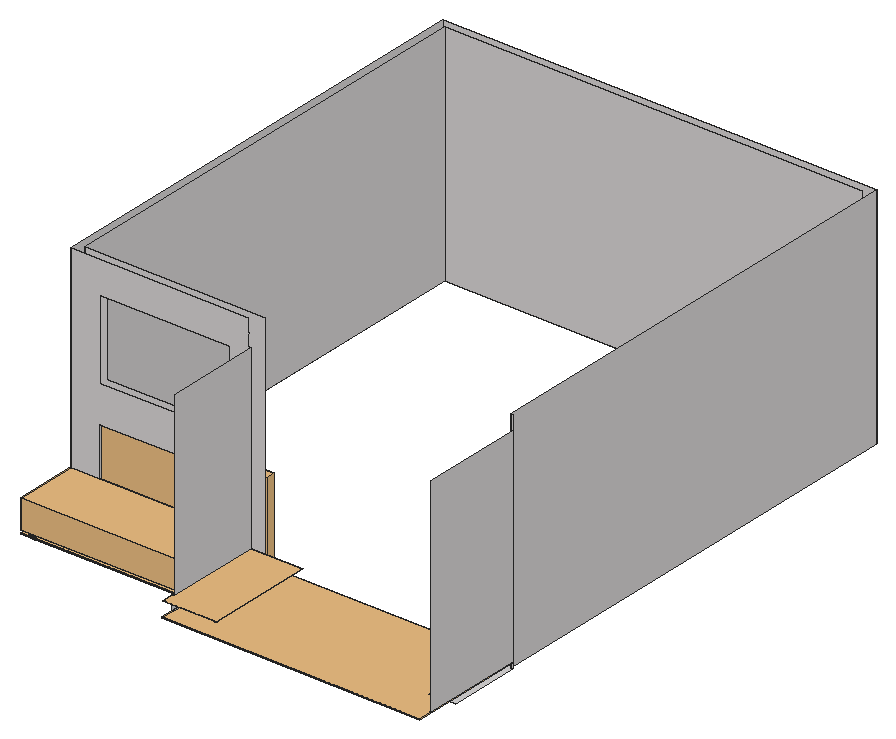
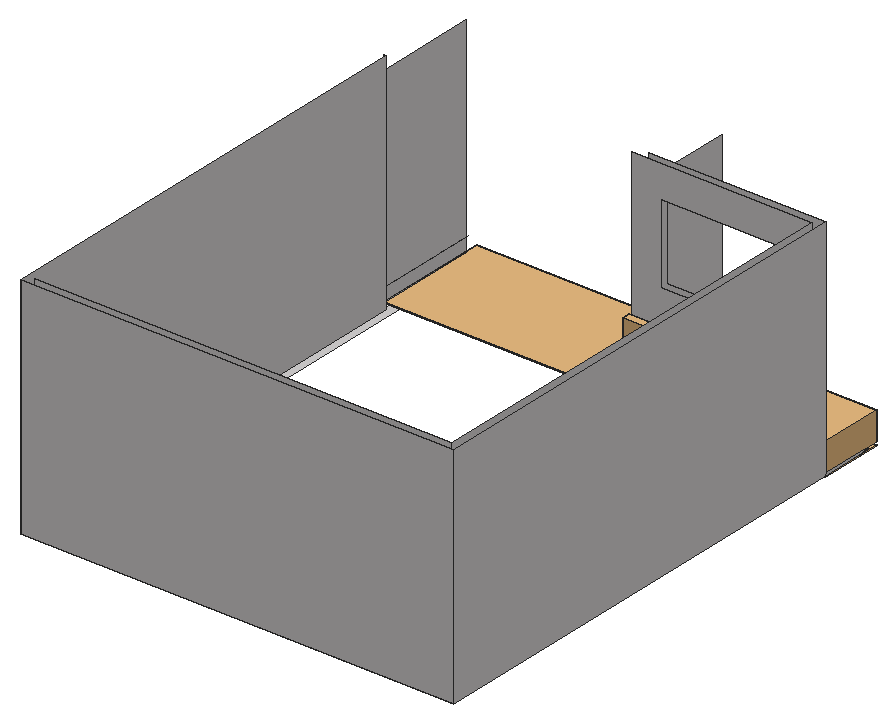
# SketchUp Ruby script. Lengths in inches.
U = 1.inch
M = Sketchup.active_model
def pt(a) = Geom::Point3d.new(a.map { |v| v * U })
def face(e, loops, mat)
  f = e.add_face(loops[0].map { |a| pt(a) })
  loops[1..].each { |l| e.add_face(l.map { |a| pt(a) }).erase! }
  f.material = f.back_material = mat if mat
  f
end
# faces: each face lists its corners as indices into pts; further lists are holes
def faces(e, pts, list, mat = nil) = list.each { |f| face(e, (f[0].is_a?(Array) ? f : [f]).map { |l| l.map { |i| pts[i] } }, mat) }
# xy, xz, yz: faces in a plane at the given z, y or x. An outline is a flat list of corners, or four numbers for a rectangle; further outlines are holes
def ring(l) = l.size == 4 ? [[l[0], l[1]], [l[2], l[1]], [l[2], l[3]], [l[0], l[3]]] : l.each_slice(2).to_a
def flat(e, list, mat, &to3) = list.each { |f| face(e, (f[0].is_a?(Array) ? f : [f]).map { |l| ring(l).map { |u, v| to3.(u, v) } }, mat) }
def xy(e, z, list, mat = nil) = flat(e, list, mat) { |x, y| [x, y, z] }
def xz(e, y, list, mat = nil) = flat(e, list, mat) { |x, z| [x, y, z] }
def yz(e, x, list, mat = nil) = flat(e, list, mat) { |y, z| [x, y, z] }
def lines(e, pts, list) = list.each { |a, b| e.add_line(pt(pts[a]), pt(pts[b])) }
# prism: a flat outline (further loops are holes) pulled along v
def prism(e, loops, v, mat = nil)
  f = face(e, loops, mat); d = Geom::Vector3d.new(v.map { |x| x * U })
  f.pushpull(f.normal.samedirection?(d) ? d.length : -d.length)
end
def box(e, o, s, mat = nil) = prism(e, [[o, [o[0] + s[0], o[1], o[2]], [o[0] + s[0], o[1] + s[1], o[2]], [o[0], o[1] + s[1], o[2]]]], [0, 0, s[2]], mat)
def at(x, y, z, deg = 0) = Geom::Transformation.translation(pt([x, y, z])) * Geom::Transformation.rotation(ORIGIN, Z_AXIS, deg.degrees)
def axes(o, x, y, z) = Geom::Transformation.new([*x, 0, *y, 0, *z, 0, *pt(o).to_a, 1])
def part(name) = M.definitions.add(name)
# library, detail: a bought-in or finely detailed component or shape, given as its bounding box
def library(name, o, s) = part(name).tap { |d| box(d.entities, o, s) }
def detail(e, o, s) = box(e.add_group.entities, o, s)
def put(e, d, t, mat = nil) = e.add_instance(d, t).tap { |i| i.material = mat if mat }
def group(e, t, mat = nil) = e.add_group.tap { |g| g.transformation = t; g.material = mat if mat }.entities
root = M.entities
M.materials.add("Outer Light - 1").color = [251, 216, 141]
M.materials.add("T METAL").color = [42, 41, 39]
M.materials.add("[Marble Carrara Floor Tile]").color = [204, 208, 219]
M.materials.add("[Quartz Light Brown]").color = [215, 212, 212]
c1 = library("Group\#10",[0,0,0],[61.75,122.25,0.25])
c2 = library("Group\#15",[-0.75,-0.75,0],[293.5,131.75,1])
c3 = library("Group\#20",[-0.5,-0.5,0],[204,72,1])
c4 = library("Group\#23",[0,0,0],[201,72,32])
c5 = library("Glass Door Sliding Door 4 Panel on 2 Tracks _ Model by Pooh",[0,0,0],[157.59,4.01,102.67])
c6 = library("Garniza_zaclona",[1.52,0,0],[127.96,8.15,78.72])
xy(root,125,[[17.76,194,201,194,201,194.5,17.77,194.5,17.54,194.51,17.3125,194.51,17.08,194.52,16.86,194.54,16.625,194.55,16.4,194.57,16.17,194.6,15.94,194.62,15.72,194.65,15.49,194.68,15.26,194.72,15.04,194.75,14.8125,194.79,14.59,194.84,14.36,194.88,14.14,194.93,13.91,194.98,13.03,195.22,12.8125,195.29,12.59,195.36,12.16,195.5,11.94,195.58,11.73,195.66,11.52,195.75,11.3,195.83,10.88,196.01,10.67,196.11,10.47,196.2,10.26,196.3,10.06,196.41,9.85,196.51,9.25,196.84,9.05,196.96,8.86,197.08,8.66,197.2,8.47,197.32,7.71,197.84,6.99,198.4,6.81,198.55,6.63,198.69,6.29,198.99,5.95,199.31,5.79,199.46,5.46,199.79,5.31,199.95,4.99,200.29,4.69,200.63,4.55,200.81,4.4,200.99,3.84,201.71,3.32,202.47,3.2,202.66,3.08,202.86,2.96,203.05,2.84,203.25,2.51,203.85,2.41,204.06,2.3,204.26,2.2,204.47,2.11,204.67,2.01,204.88,1.83,205.3,1.75,205.52,1.66,205.73,1.58,205.94,1.5,206.16,1.36,206.59,1.29,206.8125,1.22,207.03,0.98,207.91,0.93,208.14,0.88,208.36,0.84,208.59,0.79,208.8125,0.75,209.04,0.72,209.26,0.68,209.49,0.65,209.72,0.62,209.94,0.6,210.17,0.57,210.4,0.55,210.625,0.54,210.86,0.52,211.08,0.51,211.3125,0.51,211.54,0.5,211.77,0.5,266,0,266,0,211.76,0.01,211.53,0.01,211.29,0.02,211.06,0.04,210.82,0.06,210.59,0.08,210.35,0.1,210.12,0.125,209.88,0.15,209.65,0.1875,209.42,0.22,209.18,0.3,208.72,0.35,208.49,0.39,208.26,0.44,208.03,0.5,207.8,0.55,207.57,0.61,207.34,0.68,207.11,0.74,206.89,0.81,206.66,0.88,206.4375,0.96,206.21,1.03,205.99,1.11,205.77,1.2,205.55,1.28,205.33,1.46,204.89,1.56,204.68,1.65,204.46,1.75,204.25,1.86,204.04,1.96,203.83,2.18,203.41,2.3,203.2,2.41,203,2.65,202.6,2.78,202.39,2.9,202.2,3.03,202,3.17,201.8,3.3,201.61,3.4375,201.42,3.58,201.23,3.72,201.04,3.86,200.86,4.01,200.67,4.16,200.49,4.3125,200.31,4.47,200.13,4.625,199.96,4.78,199.78,4.94,199.61,5.11,199.44,5.27,199.27,5.44,199.11,5.61,198.94,5.78,198.78,5.96,198.625,6.13,198.47,6.31,198.3125,6.49,198.16,6.67,198.01,6.86,197.86,7.04,197.72,7.23,197.58,7.42,197.4375,7.61,197.3,7.8,197.17,8,197.03,8.2,196.9,8.39,196.78,8.6,196.65,9,196.41,9.2,196.3,9.41,196.18,9.83,195.96,10.04,195.86,10.25,195.75,10.46,195.65,10.68,195.56,10.89,195.46,11.33,195.28,11.55,195.2,11.77,195.11,11.99,195.03,12.21,194.96,12.4375,194.88,12.66,194.81,12.89,194.74,13.11,194.68,13.34,194.61,13.57,194.55,13.8,194.5,14.03,194.44,14.26,194.39,14.49,194.35,14.72,194.3,15.18,194.22,15.42,194.1875,15.65,194.15,15.88,194.125,16.12,194.1,16.35,194.08,16.59,194.06,16.82,194.04,17.06,194.02,17.29,194.01,17.53,194.01]],"[Quartz Light Brown]")
xy(root,126,[[0,266,3,794]],"[Marble Carrara Floor Tile]")
xy(root,126,[[17.76,194,17.53,194.01,17.29,194.01,17.06,194.02,16.82,194.04,16.59,194.06,16.35,194.08,16.12,194.1,15.88,194.125,15.65,194.15,15.42,194.1875,15.18,194.22,14.72,194.3,14.49,194.35,14.26,194.39,14.03,194.44,13.8,194.5,13.57,194.55,13.34,194.61,13.11,194.68,12.89,194.74,12.66,194.81,12.4375,194.88,12.21,194.96,11.99,195.03,11.77,195.11,11.55,195.2,11.33,195.28,10.89,195.46,10.68,195.56,10.46,195.65,10.25,195.75,10.04,195.86,9.83,195.96,9.41,196.18,9.2,196.3,9,196.41,8.6,196.65,8.39,196.78,8.2,196.9,8,197.03,7.8,197.17,7.61,197.3,7.42,197.4375,7.23,197.58,7.04,197.72,6.86,197.86,6.67,198.01,6.49,198.16,6.31,198.3125,6.13,198.47,5.96,198.625,5.78,198.78,5.61,198.94,5.44,199.11,5.27,199.27,5.11,199.44,4.94,199.61,4.78,199.78,4.625,199.96,4.47,200.13,4.3125,200.31,4.16,200.49,4.01,200.67,3.86,200.86,3.72,201.04,3.58,201.23,3.4375,201.42,3.3,201.61,3.17,201.8,3.03,202,2.9,202.2,2.78,202.39,2.65,202.6,2.41,203,2.3,203.2,2.18,203.41,1.96,203.83,1.86,204.04,1.75,204.25,1.65,204.46,1.56,204.68,1.46,204.89,1.28,205.33,1.2,205.55,1.11,205.77,1.03,205.99,0.96,206.21,0.88,206.4375,0.81,206.66,0.74,206.89,0.68,207.11,0.61,207.34,0.55,207.57,0.5,207.8,0.44,208.03,0.39,208.26,0.35,208.49,0.3,208.72,0.22,209.18,0.1875,209.42,0.15,209.65,0.125,209.88,0.1,210.12,0.08,210.35,0.06,210.59,0.04,210.82,0.02,211.06,0.01,211.29,0.01,211.53,0,211.76,0,266,0.5,266,0.5,211.77,0.51,211.54,0.51,211.3125,0.52,211.08,0.54,210.86,0.55,210.625,0.57,210.4,0.6,210.17,0.62,209.94,0.65,209.72,0.68,209.49,0.72,209.26,0.75,209.04,0.79,208.8125,0.84,208.59,0.88,208.36,0.93,208.14,0.98,207.91,1.22,207.03,1.29,206.8125,1.36,206.59,1.5,206.16,1.58,205.94,1.66,205.73,1.75,205.52,1.83,205.3,2.01,204.88,2.11,204.67,2.2,204.47,2.3,204.26,2.41,204.06,2.51,203.85,2.84,203.25,2.96,203.05,3.08,202.86,3.2,202.66,3.32,202.47,3.84,201.71,4.4,200.99,4.55,200.81,4.69,200.63,4.99,200.29,5.31,199.95,5.46,199.79,5.79,199.46,5.95,199.31,6.29,198.99,6.63,198.69,6.81,198.55,6.99,198.4,7.71,197.84,8.47,197.32,8.66,197.2,8.86,197.08,9.05,196.96,9.25,196.84,9.85,196.51,10.06,196.41,10.26,196.3,10.47,196.2,10.67,196.11,10.88,196.01,11.3,195.83,11.52,195.75,11.73,195.66,11.94,195.58,12.16,195.5,12.59,195.36,12.8125,195.29,13.03,195.22,13.91,194.98,14.14,194.93,14.36,194.88,14.59,194.84,14.8125,194.79,15.04,194.75,15.26,194.72,15.49,194.68,15.72,194.65,15.94,194.62,16.17,194.6,16.4,194.57,16.625,194.55,16.86,194.54,17.08,194.52,17.3125,194.51,17.54,194.51,17.77,194.5,201,194.5,201,194],[483,194,483,785,9,785,9,266,0,266,0,794,492,794,492,275,495,275,495,194],[201,194,201,266,180,266,180,275,213,275,213,194],[9,266,33,275]],"[Quartz Light Brown]")
xy(root,129,[[17.76,194,201,194,201,197,17.8,197,17.61,197.01,17.41,197.01,17.21,197.02,17.02,197.03,16.82,197.05,16.63,197.0625,16.43,197.08,16.24,197.1,16.04,197.13,15.85,197.16,15.65,197.18,15.46,197.22,15.27,197.25,15.07,197.29,14.5,197.41,14.12,197.51,13.93,197.5625,13.74,197.62,13.55,197.67,13.36,197.73,13.18,197.8,12.99,197.86,12.81,197.93,12.44,198.07,12.26,198.14,11.54,198.46,11.37,198.55,11.19,198.63,11.02,198.73,10.84,198.82,10.67,198.91,10.16,199.21,10,199.3125,9.83,199.42,9.67,199.53,9.5,199.64,9.18,199.86,9.03,199.98,8.71,200.22,8.56,200.34,8.41,200.47,8.26,200.59,7.96,200.85,7.82,200.99,7.67,201.12,7.53,201.26,7.39,201.39,7.26,201.53,7.12,201.67,6.99,201.82,6.85,201.96,6.59,202.26,6.47,202.41,6.34,202.56,6.22,202.71,5.98,203.03,5.86,203.18,5.64,203.5,5.53,203.67,5.42,203.83,5.3125,204,5.21,204.16,4.91,204.67,4.82,204.84,4.73,205.02,4.63,205.19,4.55,205.37,4.46,205.54,4.14,206.26,4.07,206.44,3.93,206.81,3.86,206.99,3.8,207.18,3.73,207.36,3.67,207.55,3.62,207.74,3.5625,207.93,3.51,208.12,3.41,208.5,3.29,209.07,3.25,209.27,3.22,209.46,3.18,209.65,3.16,209.85,3.13,210.04,3.1,210.24,3.08,210.43,3.0625,210.63,3.05,210.82,3.03,211.02,3.02,211.21,3.01,211.41,3.01,211.61,3,211.8,3,266,0,266,0,211.76,0.01,211.53,0.01,211.29,0.02,211.06,0.04,210.82,0.06,210.59,0.08,210.35,0.1,210.12,0.125,209.88,0.15,209.65,0.1875,209.42,0.22,209.18,0.3,208.72,0.35,208.49,0.39,208.26,0.44,208.03,0.5,207.8,0.55,207.57,0.61,207.34,0.68,207.11,0.74,206.89,0.81,206.66,0.88,206.4375,0.96,206.21,1.03,205.99,1.11,205.77,1.2,205.55,1.28,205.33,1.46,204.89,1.56,204.68,1.65,204.46,1.75,204.25,1.86,204.04,1.96,203.83,2.18,203.41,2.3,203.2,2.41,203,2.65,202.6,2.78,202.39,2.9,202.2,3.03,202,3.17,201.8,3.3,201.61,3.4375,201.42,3.58,201.23,3.72,201.04,3.86,200.86,4.01,200.67,4.16,200.49,4.3125,200.31,4.47,200.13,4.625,199.96,4.78,199.78,4.94,199.61,5.11,199.44,5.27,199.27,5.44,199.11,5.61,198.94,5.78,198.78,5.96,198.625,6.13,198.47,6.31,198.3125,6.49,198.16,6.67,198.01,6.86,197.86,7.04,197.72,7.23,197.58,7.42,197.4375,7.61,197.3,7.8,197.17,8,197.03,8.2,196.9,8.39,196.78,8.6,196.65,9,196.41,9.2,196.3,9.41,196.18,9.83,195.96,10.04,195.86,10.25,195.75,10.46,195.65,10.68,195.56,10.89,195.46,11.33,195.28,11.55,195.2,11.77,195.11,11.99,195.03,12.21,194.96,12.4375,194.88,12.66,194.81,12.89,194.74,13.11,194.68,13.34,194.61,13.57,194.55,13.8,194.5,14.03,194.44,14.26,194.39,14.49,194.35,14.72,194.3,15.18,194.22,15.42,194.1875,15.65,194.15,15.88,194.125,16.12,194.1,16.35,194.08,16.59,194.06,16.82,194.04,17.06,194.02,17.29,194.01,17.53,194.01]],"[Quartz Light Brown]")
xz(root,266,[[0,125,0.5,126],[0,126,3,129],[[0,126,33,126,33,216,180,216,180,126,201,126,201,132,202,132,202,133,201,133,201,150,201.75,150,201.75,149.75,202.25,149.75,202.25,150,204,150,204,354,202.25,354,202.25,354.25,201.75,354.25,201.75,354,201,354,201,368,202,368,202,369,201,369,201,384,0,384],[33,257.9,180,348]]],"[Quartz Light Brown]")
xz(root,275,[[[9,126,9,384,213,384,213,126,180,126,180,216,33,216,33,126],[33,257.9,180,348]],[492,126,492,150,495,150,495,133,494,133,494,132,495,132,495,126],[492,150,492,384,495,384,495,369,494,369,494,368,495,368,495,150]],"[Quartz Light Brown]")
xz(root,785,[[9,126,483,384]],"[Quartz Light Brown]")
xz(root,794,[[0,126,492,384]],"[Quartz Light Brown]")
yz(root,0,[[211.76,126,212,129],[212,126,266,129],[266,126,794,384]],"[Quartz Light Brown]")
yz(root,0.01,[[211.29,126,211.53,129]],"[Quartz Light Brown]")
yz(root,0.5,[[211.77,125,212,126],[212,125,266,126]],"[Quartz Light Brown]")
yz(root,0.51,[[211.3125,125,211.54,126]],"[Quartz Light Brown]")
yz(root,3,[[211.8,126,212,129],[212,126,266,129]],"[Quartz Light Brown]")
yz(root,3.01,[[211.41,126,211.61,129]],"[Quartz Light Brown]")
yz(root,9,[[275,126,785,384]],"[Quartz Light Brown]")
yz(root,33,[[266,126,275,216]],"[Quartz Light Brown]")
yz(root,180,[[266,126,275,216]],"[Quartz Light Brown]")
yz(root,201,[[158,133,266,150]],"[Quartz Light Brown]")
yz(root,201.75,[[158,149.75,266,150]],"[Quartz Light Brown]")
yz(root,202,[[158,132,266,133]],"[Quartz Light Brown]")
yz(root,202.25,[[158,149.75,266,150]],"[Quartz Light Brown]")
yz(root,204,[[158,150,266,354]],"[Quartz Light Brown]")
yz(root,492,[[275,126,794,384]],"[Quartz Light Brown]")
yz(root,494,[[158,132,275,133]],"[Quartz Light Brown]")
yz(root,495,[[158,133,275,368]],"[Quartz Light Brown]")
p = [[8.09,197.58,126],[8.09,197.58,125],[8.28,197.45,125],[8.28,197.45,126],[7.9,197.71,126],[7.9,197.71,125],
  [7.71,197.84,126],[7.71,197.84,125],[7.53,197.98,126],[7.53,197.98,125],[7.35,198.12,126],[7.35,198.12,125],
  [7.17,198.26,126],[7.17,198.26,125],[6.99,198.4,126],[6.99,198.4,125],[6.81,198.55,126],[6.81,198.55,125],
  [6.63,198.69,126],[6.63,198.69,125],[6.46,198.84,126],[6.46,198.84,125],[6.29,198.99,126],[6.29,198.99,125],
  [6.12,199.15,126],[6.12,199.15,125],[5.95,199.31,126],[5.95,199.31,125],[5.79,199.46,126],[5.79,199.46,125],
  [5.625,199.625,126],[5.625,199.625,125],[5.46,199.79,126],[5.46,199.79,125],[5.31,199.95,126],[5.31,199.95,125],
  [5.15,200.12,126],[5.15,200.12,125],[4.99,200.29,126],[4.99,200.29,125],[4.84,200.46,126],[4.84,200.46,125],
  [4.69,200.63,126],[4.69,200.63,125],[4.55,200.81,126],[4.55,200.81,125],[4.4,200.99,126],[4.4,200.99,125],
  [4.26,201.17,126],[4.26,201.17,125],[4.12,201.35,126],[4.12,201.35,125],[3.98,201.53,126],[3.98,201.53,125],
  [3.84,201.71,126],[3.84,201.71,125],[3.71,201.9,126],[3.71,201.9,125],[3.58,202.09,126],[3.58,202.09,125],
  [3.45,202.28,126],[3.45,202.28,125],[3.32,202.47,126],[3.32,202.47,125],[3.2,202.66,126],[3.2,202.66,125],
  [3.08,202.86,126],[3.08,202.86,125],[2.96,203.05,126],[2.96,203.05,125],[2.84,203.25,126],[2.84,203.25,125],
  [2.73,203.45,126],[2.73,203.45,125],[2.62,203.65,126],[2.62,203.65,125],[2.51,203.85,126],[2.51,203.85,125],
  [2.41,204.06,126],[2.41,204.06,125],[2.3,204.26,126],[2.3,204.26,125],[2.2,204.47,126],[2.2,204.47,125],
  [2.11,204.67,126],[2.11,204.67,125],[2.01,204.88,126],[2.01,204.88,125],[1.92,205.09,126],[1.92,205.09,125],
  [1.83,205.3,126],[1.83,205.3,125],[1.75,205.52,126],[1.75,205.52,125],[1.66,205.73,126],[1.66,205.73,125],
  [1.58,205.94,126],[1.58,205.94,125],[1.5,206.16,126],[1.5,206.16,125],[1.43,206.375,126],[1.43,206.375,125],
  [1.36,206.59,126],[1.36,206.59,125],[1.29,206.8125,126],[1.29,206.8125,125],[1.22,207.03,126],[1.22,207.03,125],
  [1.16,207.25,126],[1.16,207.25,125],[1.1,207.47,126],[1.1,207.47,125],[1.04,207.69,126],[1.04,207.69,125],
  [0.98,207.91,126],[0.98,207.91,125],[0.93,208.14,126],[0.93,208.14,125],[0.88,208.36,126],[0.88,208.36,125],
  [0.84,208.59,126],[0.84,208.59,125],[0.79,208.8125,126],[0.79,208.8125,125],[0.75,209.04,126],[0.75,209.04,125],
  [0.72,209.26,126],[0.72,209.26,125],[0.68,209.49,126],[0.68,209.49,125],[0.65,209.72,126],[0.65,209.72,125],
  [0.62,209.94,126],[0.62,209.94,125],[0.6,210.17,126],[0.6,210.17,125],[0.57,210.4,126],[0.57,210.4,125],
  [0.55,210.625,126],[0.55,210.625,125],[0.54,210.86,126],[0.54,210.86,125],[0.52,211.08,126],[0.52,211.08,125],
  [0.51,211.3125,126],[0.51,211.3125,125],[0.5,211.77,126],[0.5,211.77,125],[0.51,211.54,125],[0.51,211.54,126],
  [7.42,197.4375,126],[7.42,197.4375,129],[7.23,197.58,129],[7.23,197.58,126],[14.5,197.41,126],[14.31,197.46,126],
  [14.31,197.46,129],[14.5,197.41,129],[14.69,197.37,126],[14.69,197.37,129],[14.12,197.51,126],[13.93,197.5625,126],
  [13.93,197.5625,129],[14.12,197.51,129],[7.04,197.72,129],[7.04,197.72,126],[13.74,197.62,126],[13.55,197.67,126],
  [13.55,197.67,129],[13.74,197.62,129],[6.86,197.86,129],[6.86,197.86,126],[13.36,197.73,126],[13.18,197.8,126],
  [13.18,197.8,129],[13.36,197.73,129],[12.99,197.86,126],[12.99,197.86,129],[6.67,198.01,129],[6.67,198.01,126],
  [12.81,197.93,126],[12.625,198,126],[12.625,198,129],[12.81,197.93,129],[6.49,198.16,129],[6.49,198.16,126],
  [12.44,198.07,126],[12.44,198.07,129],[12.26,198.14,126],[12.08,198.22,126],[12.08,198.22,129],[12.26,198.14,129],
  [6.31,198.3125,129],[6.31,198.3125,126],[11.9,198.3,126],[11.9,198.3,129],[6.13,198.47,129],[6.13,198.47,126],
  [11.72,198.38,126],[11.72,198.38,129],[11.54,198.46,126],[11.54,198.46,129],[5.96,198.625,129],[5.96,198.625,126],
  [11.37,198.55,126],[11.19,198.63,126],[11.19,198.63,129],[11.37,198.55,129],[5.78,198.78,129],[5.78,198.78,126],
  [11.02,198.73,126],[11.02,198.73,129],[10.84,198.82,126],[10.84,198.82,129],[5.61,198.94,129],[5.61,198.94,126],
  [10.67,198.91,126],[10.67,198.91,129],[5.44,199.11,129],[5.44,199.11,126],[10.5,199.01,126],[10.5,199.01,129],
  [10.33,199.11,126],[10.33,199.11,129],[5.27,199.27,129],[5.27,199.27,126],[10.16,199.21,126],[10.16,199.21,129],
  [10,199.3125,126],[10,199.3125,129],[5.11,199.44,129],[5.11,199.44,126],[9.83,199.42,126],[9.83,199.42,129],
  [4.94,199.61,129],[4.94,199.61,126],[9.67,199.53,126],[9.67,199.53,129],[9.5,199.64,126],[9.5,199.64,129],
  [4.78,199.78,129],[4.78,199.78,126],[9.34,199.75,126],[9.34,199.75,129],[4.625,199.96,129],[4.625,199.96,126],
  [9.18,199.86,126],[9.18,199.86,129],[9.03,199.98,126],[9.03,199.98,129],[4.47,200.13,129],[4.47,200.13,126],
  [8.87,200.1,126],[8.87,200.1,129],[4.3125,200.31,129],[4.3125,200.31,126],[8.71,200.22,126],[8.71,200.22,129],
  [8.56,200.34,126],[8.56,200.34,129],[4.16,200.49,129],[4.16,200.49,126],[8.41,200.47,126],[8.41,200.47,129],
  [4.01,200.67,129],[4.01,200.67,126],[8.26,200.59,126],[8.26,200.59,129],[8.11,200.72,126],[8.11,200.72,129],
  [3.86,200.86,129],[3.86,200.86,126],[7.96,200.85,126],[7.96,200.85,129],[3.72,201.04,129],[3.72,201.04,126],
  [7.82,200.99,126],[7.82,200.99,129],[3.58,201.23,129],[3.58,201.23,126],[7.67,201.12,126],[7.67,201.12,129],
  [7.53,201.26,126],[7.53,201.26,129],[3.4375,201.42,129],[3.4375,201.42,126],[7.39,201.39,126],[7.39,201.39,129],
  [3.3,201.61,129],[3.3,201.61,126],[7.26,201.53,126],[7.26,201.53,129],[7.12,201.67,126],[7.12,201.67,129],
  [3.17,201.8,129],[3.17,201.8,126],[6.99,201.82,126],[6.99,201.82,129],[3.03,202,129],[3.03,202,126],
  [6.85,201.96,126],[6.85,201.96,129],[2.9,202.2,129],[2.9,202.2,126],[6.72,202.11,126],[6.72,202.11,129],
  [6.59,202.26,126],[6.59,202.26,129],[2.78,202.39,129],[2.78,202.39,126],[6.47,202.41,126],[6.47,202.41,129],
  [2.65,202.6,129],[2.65,202.6,126],[6.34,202.56,126],[6.34,202.56,129],[2.53,202.8,129],[2.53,202.8,126],
  [6.22,202.71,126],[6.22,202.71,129],[6.1,202.87,126],[6.1,202.87,129],[2.41,203,129],[2.41,203,126],
  [5.98,203.03,126],[5.98,203.03,129],[2.3,203.2,129],[2.3,203.2,126],[5.86,203.18,126],[5.86,203.18,129],
  [2.18,203.41,129],[2.18,203.41,126],[5.75,203.34,126],[5.75,203.34,129],[5.64,203.5,126],[5.64,203.5,129],
  [2.07,203.62,129],[2.07,203.62,126],[5.53,203.67,126],[5.53,203.67,129],[1.96,203.83,129],[1.96,203.83,126],
  [5.42,203.83,126],[5.42,203.83,129],[1.86,204.04,129],[1.86,204.04,126],[5.3125,204,126],[5.3125,204,129],
  [1.75,204.25,129],[1.75,204.25,126],[5.21,204.16,126],[5.21,204.16,129],[5.11,204.33,126],[5.11,204.33,129],
  [1.65,204.46,129],[1.65,204.46,126],[5.01,204.5,126],[5.01,204.5,129],[1.56,204.68,129],[1.56,204.68,126],
  [4.91,204.67,126],[4.91,204.67,129],[1.46,204.89,129],[1.46,204.89,126],[4.82,204.84,126],[4.82,204.84,129],
  [4.73,205.02,126],[4.73,205.02,129],[1.37,205.11,129],[1.37,205.11,126],[4.63,205.19,126],[4.63,205.19,129],
  [1.28,205.33,129],[1.28,205.33,126],[4.55,205.37,126],[4.55,205.37,129],[1.2,205.55,129],[1.2,205.55,126],
  [4.46,205.54,126],[4.46,205.54,129],[1.11,205.77,129],[1.11,205.77,126],[4.38,205.72,126],[4.38,205.72,129],
  [4.3,205.9,126],[4.3,205.9,129],[1.03,205.99,129],[1.03,205.99,126],[4.22,206.08,126],[4.22,206.08,129],
  [0.96,206.21,129],[0.96,206.21,126],[4.14,206.26,126],[4.14,206.26,129],[0.88,206.4375,129],[0.88,206.4375,126],
  [4.07,206.44,126],[4.07,206.44,129],[0.81,206.66,129],[0.81,206.66,126],[4,206.625,126],[4,206.625,129],
  [3.93,206.81,126],[3.93,206.81,129],[0.74,206.89,129],[0.74,206.89,126],[3.86,206.99,126],[3.86,206.99,129],
  [0.68,207.11,129],[0.68,207.11,126],[3.8,207.18,126],[3.8,207.18,129],[0.61,207.34,129],[0.61,207.34,126],
  [3.73,207.36,126],[3.73,207.36,129],[0.55,207.57,129],[0.55,207.57,126],[3.67,207.55,126],[3.67,207.55,129],
  [0.5,207.8,129],[0.5,207.8,126],[3.62,207.74,126],[3.62,207.74,129],[3.5625,207.93,126],[3.5625,207.93,129],
  [0.44,208.03,129],[0.44,208.03,126],[3.51,208.12,126],[3.51,208.12,129],[0.39,208.26,129],[0.39,208.26,126],
  [3.46,208.31,126],[3.46,208.31,129],[0.35,208.49,129],[0.35,208.49,126],[3.41,208.5,126],[3.41,208.5,129],
  [0.3,208.72,129],[0.3,208.72,126],[3.37,208.69,126],[3.37,208.69,129],[0.26,208.95,129],[0.26,208.95,126],
  [3.33,208.88,126],[3.33,208.88,129],[3.29,209.07,126],[3.29,209.07,129],[0.22,209.18,129],[0.22,209.18,126],
  [3.25,209.27,126],[3.25,209.27,129],[0.1875,209.42,129],[0.1875,209.42,126],[3.22,209.46,126],[3.22,209.46,129],
  [0.15,209.65,129],[0.15,209.65,126],[3.18,209.65,126],[3.18,209.65,129],[0.125,209.88,129],[0.125,209.88,126],
  [3.16,209.85,126],[3.16,209.85,129],[3.13,210.04,126],[3.13,210.04,129],[0.1,210.12,129],[0.1,210.12,126],
  [3.1,210.24,126],[3.1,210.24,129],[0.08,210.35,129],[0.08,210.35,126],[3.08,210.43,126],[3.08,210.43,129],
  [0.06,210.59,129],[0.06,210.59,126],[3.0625,210.63,126],[3.0625,210.63,129],[0.04,210.82,129],[0.04,210.82,126],
  [3.05,210.82,126],[3.05,210.82,129],[0.02,211.06,129],[0.02,211.06,126],[3.03,211.02,126],[3.03,211.02,129],
  [3.02,211.21,126],[3.02,211.21,129],[0.01,211.29,129],[0.01,211.29,126],[3.01,211.41,126],[3.01,211.41,129],
  [0.01,211.53,126],[0.01,211.53,129],[0,211.76,129],[0,211.76,126],[3.01,211.61,126],[3,211.8,126],
  [3,211.8,129],[3.01,211.61,129],[492,158,150],[492,275,150]]
faces(root,p,[[0,1,2,3],[4,5,1,0],[6,7,5,4],[8,9,7,6],[10,11,9,8],[12,13,11,10],[14,15,13,12],[16,17,15,14],
  [18,19,17,16],[20,21,19,18],[22,23,21,20],[24,25,23,22],[26,27,25,24],[28,29,27,26],[30,31,29,28],[32,33,31,30],
  [34,35,33,32],[36,37,35,34],[38,39,37,36],[40,41,39,38],[42,43,41,40],[44,45,43,42],[46,47,45,44],[48,49,47,46],
  [50,51,49,48],[52,53,51,50],[54,55,53,52],[56,57,55,54],[58,59,57,56],[60,61,59,58],[62,63,61,60],[64,65,63,62],
  [66,67,65,64],[68,69,67,66],[70,71,69,68],[72,73,71,70],[74,75,73,72],[76,77,75,74],[78,79,77,76],[80,81,79,78],
  [82,83,81,80],[84,85,83,82],[86,87,85,84],[88,89,87,86],[90,91,89,88],[92,93,91,90],[94,95,93,92],[96,97,95,94],
  [98,99,97,96],[100,101,99,98],[102,103,101,100],[104,105,103,102],[106,107,105,104],[108,109,107,106],[110,111,109,108],[112,113,111,110],
  [114,115,113,112],[116,117,115,114],[118,119,117,116],[120,121,119,118],[122,123,121,120],[124,125,123,122],[126,127,125,124],[128,129,127,126],
  [130,131,129,128],[132,133,131,130],[134,135,133,132],[136,137,135,134],[138,139,137,136],[140,141,139,138],[142,143,141,140],[144,145,143,142],
  [146,147,148,149],[150,151,152,153],[154,155,156,157],[158,154,157,159],[160,161,162,163],[155,160,163,156],[153,152,164,165],[166,167,168,169],
  [161,166,169,162],[165,164,170,171],[172,173,174,175],[167,172,175,168],[173,176,177,174],[171,170,178,179],[180,181,182,183],[176,180,183,177],
  [179,178,184,185],[181,186,187,182],[188,189,190,191],[186,188,191,187],[185,184,192,193],[189,194,195,190],[193,192,196,197],[194,198,199,195],
  [198,200,201,199],[197,196,202,203],[204,205,206,207],[200,204,207,201],[203,202,208,209],[205,210,211,206],[210,212,213,211],[209,208,214,215],
  [212,216,217,213],[215,214,218,219],[216,220,221,217],[220,222,223,221],[219,218,224,225],[222,226,227,223],[226,228,229,227],[225,224,230,231],
  [228,232,233,229],[231,230,234,235],[232,236,237,233],[236,238,239,237],[235,234,240,241],[238,242,243,239],[241,240,244,245],[242,246,247,243],
  [246,248,249,247],[245,244,250,251],[248,252,253,249],[251,250,254,255],[252,256,257,253],[256,258,259,257],[255,254,260,261],[258,262,263,259],
  [261,260,264,265],[262,266,267,263],[266,268,269,267],[265,264,270,271],[268,272,273,269],[271,270,274,275],[272,276,277,273],[275,274,278,279],
  [276,280,281,277],[280,282,283,281],[279,278,284,285],[282,286,287,283],[285,284,288,289],[286,290,291,287],[290,292,293,291],[289,288,294,295],
  [292,296,297,293],[295,294,298,299],[296,300,301,297],[299,298,302,303],[300,304,305,301],[304,306,307,305],[303,302,308,309],[306,310,311,307],
  [309,308,312,313],[310,314,315,311],[313,312,316,317],[314,318,319,315],[318,320,321,319],[317,316,322,323],[320,324,325,321],[323,322,326,327],
  [324,328,329,325],[327,326,330,331],[328,332,333,329],[332,334,335,333],[331,330,336,337],[334,338,339,335],[337,336,340,341],[338,342,343,339],
  [341,340,344,345],[342,346,347,343],[345,344,348,349],[346,350,351,347],[350,352,353,351],[349,348,354,355],[352,356,357,353],[355,354,358,359],
  [356,360,361,357],[359,358,362,363],[360,364,365,361],[364,366,367,365],[363,362,368,369],[366,370,371,367],[369,368,372,373],[370,374,375,371],
  [373,372,376,377],[374,378,379,375],[377,376,380,381],[378,382,383,379],[382,384,385,383],[381,380,386,387],[384,388,389,385],[387,386,390,391],
  [388,392,393,389],[391,390,394,395],[392,396,397,393],[395,394,398,399],[396,400,401,397],[400,402,403,401],[399,398,404,405],[402,406,407,403],
  [405,404,408,409],[406,410,411,407],[409,408,412,413],[410,414,415,411],[413,412,416,417],[414,418,419,415],[417,416,420,421],[418,422,423,419],
  [422,424,425,423],[421,420,426,427],[424,428,429,425],[427,426,430,431],[428,432,433,429],[431,430,434,435],[432,436,437,433],[435,434,438,439],
  [436,440,441,437],[439,438,442,443],[440,444,445,441],[444,446,447,445],[443,442,448,449],[446,450,451,447],[449,448,452,453],[450,454,455,451],
  [453,452,456,457],[454,458,459,455],[457,456,460,461],[458,462,463,459],[462,464,465,463],[461,460,466,467],[464,468,469,465],[467,466,470,471],
  [468,472,473,469],[471,470,474,475],[472,476,477,473],[475,474,478,479],[476,480,481,477],[479,478,482,483],[480,484,485,481],[484,486,487,485],
  [483,482,488,489],[486,490,491,487],[492,493,494,495],[496,497,498,499]],"[Quartz Light Brown]")
lines(root,p,[[500,501]])
put(root,c1,at(201.75,143.75,149.75),"Outer Light - 1")
put(root,c2,at(202,144,132),"Outer Light - 1")
put(root,c3,at(0.5,194.5,125),"Outer Light - 1")
put(root,c4,at(0,194,129),"T METAL")
put(root,c5,axes([33,267,126],[0.93279,0,0],[0,1,0],[0,0,0.87661]),"[Quartz Light Brown]")
put(root,c6,axes([9,277.55,125.89],[1.58151,0,0],[0,1.1771,0],[0,0,1.20432]))
